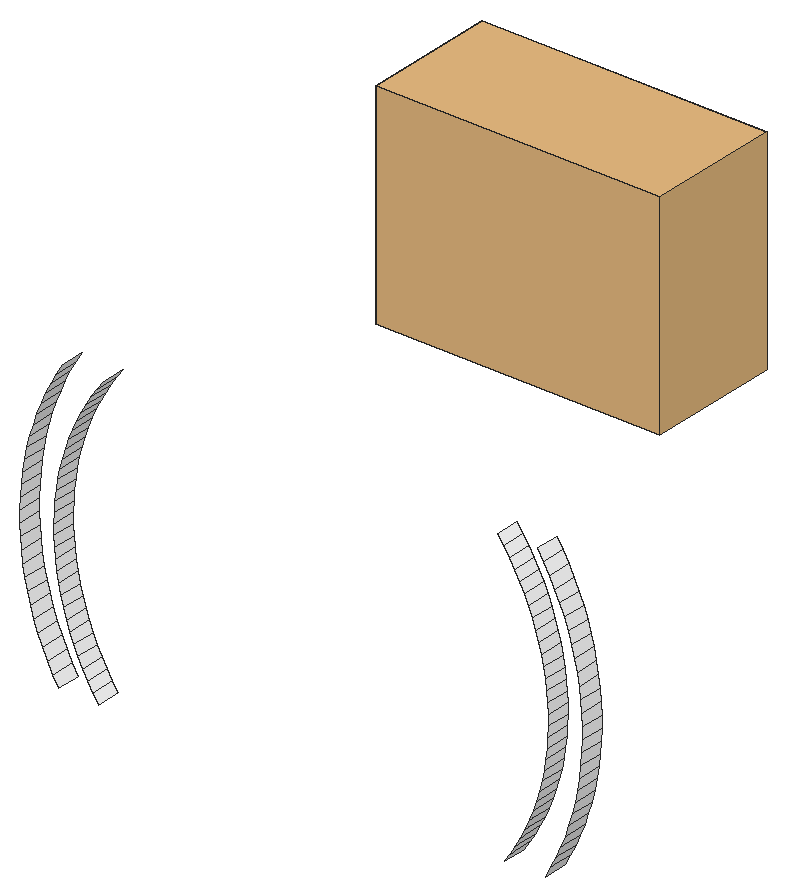
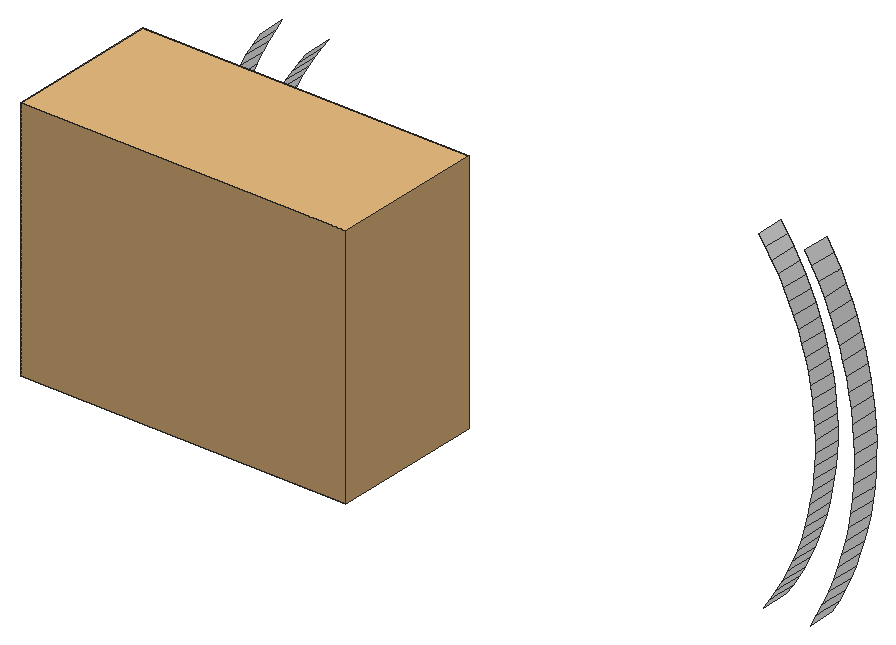
# SketchUp Ruby script. Lengths in inches.
U = 1.inch
M = Sketchup.active_model
def pt(a) = Geom::Point3d.new(a.map { |v| v * U })
def face(e, loops, mat)
  f = e.add_face(loops[0].map { |a| pt(a) })
  loops[1..].each { |l| e.add_face(l.map { |a| pt(a) }).erase! }
  f.material = f.back_material = mat if mat
  f
end
# faces: each face lists its corners as indices into pts; further lists are holes
def faces(e, pts, list, mat = nil) = list.each { |f| face(e, (f[0].is_a?(Array) ? f : [f]).map { |l| l.map { |i| pts[i] } }, mat) }
# xy, xz, yz: faces in a plane at the given z, y or x. An outline is a flat list of corners, or four numbers for a rectangle; further outlines are holes
def ring(l) = l.size == 4 ? [[l[0], l[1]], [l[2], l[1]], [l[2], l[3]], [l[0], l[3]]] : l.each_slice(2).to_a
def flat(e, list, mat, &to3) = list.each { |f| face(e, (f[0].is_a?(Array) ? f : [f]).map { |l| ring(l).map { |u, v| to3.(u, v) } }, mat) }
def xy(e, z, list, mat = nil) = flat(e, list, mat) { |x, y| [x, y, z] }
def xz(e, y, list, mat = nil) = flat(e, list, mat) { |x, z| [x, y, z] }
def yz(e, x, list, mat = nil) = flat(e, list, mat) { |y, z| [x, y, z] }
def lines(e, pts, list) = list.each { |a, b| e.add_line(pt(pts[a]), pt(pts[b])) }
# prism: a flat outline (further loops are holes) pulled along v
def prism(e, loops, v, mat = nil)
  f = face(e, loops, mat); d = Geom::Vector3d.new(v.map { |x| x * U })
  f.pushpull(f.normal.samedirection?(d) ? d.length : -d.length)
end
def box(e, o, s, mat = nil) = prism(e, [[o, [o[0] + s[0], o[1], o[2]], [o[0] + s[0], o[1] + s[1], o[2]], [o[0], o[1] + s[1], o[2]]]], [0, 0, s[2]], mat)
def at(x, y, z, deg = 0) = Geom::Transformation.translation(pt([x, y, z])) * Geom::Transformation.rotation(ORIGIN, Z_AXIS, deg.degrees)
def axes(o, x, y, z) = Geom::Transformation.new([*x, 0, *y, 0, *z, 0, *pt(o).to_a, 1])
def part(name) = M.definitions.add(name)
# library, detail: a bought-in or finely detailed component or shape, given as its bounding box
def library(name, o, s) = part(name).tap { |d| box(d.entities, o, s) }
def detail(e, o, s) = box(e.add_group.entities, o, s)
def put(e, d, t, mat = nil) = e.add_instance(d, t).tap { |i| i.material = mat if mat }
def group(e, t, mat = nil) = e.add_group.tap { |g| g.transformation = t; g.material = mat if mat }.entities
root = M.entities
M.materials.add("Leather White 002 15.0cm").color = [255, 255, 255]
c1 = library("Window Crafter Awning",[0,-9.5,0],[24,11.27,18])
yz(root,12.9,[[48.93,201.61,50.93,202.49]],"Leather White 002 15.0cm")
yz(root,57.52,[[48.93,201.78,50.93,202.77]],"Leather White 002 15.0cm")
p = [[12.79,50.93,191.04],[13.27,50.93,190.17],[13.27,48.93,190.17],[12.79,48.93,191.04],[16.69,50.93,190.15],[16.21,50.93,190.875],
  [16.21,48.93,190.875],[16.69,48.93,190.15],[51.47,50.93,191.06],[50.99,50.93,190.33],[50.99,48.93,190.33],[51.47,48.93,191.06],
  [54.41,50.93,190.39],[54.88,50.93,191.26],[54.88,48.93,191.26],[54.41,48.93,190.39],[15.75,50.93,191.62],[15.75,48.93,191.62],
  [12.34,50.93,191.93],[12.34,48.93,191.93],[51.91,50.93,191.81],[51.91,48.93,191.81],[55.32,50.93,192.15],[55.32,48.93,192.15],
  [15.32,50.93,192.39],[15.32,48.93,192.39],[52.33,50.93,192.58],[52.33,48.93,192.58],[11.93,50.93,192.84],[11.93,48.93,192.84],
  [55.72,50.93,193.0625],[55.72,48.93,193.0625],[14.93,50.93,193.17],[14.93,48.93,193.17],[52.72,50.93,193.36],[52.72,48.93,193.36],
  [11.56,50.93,193.76],[11.56,48.93,193.76],[56.08,50.93,193.99],[56.08,48.93,193.99],[14.57,50.93,193.96],[14.57,48.93,193.96],
  [53.07,50.93,194.16],[53.07,48.93,194.16],[11.23,50.93,194.7],[11.23,48.93,194.7],[14.24,50.93,194.78],[14.24,48.93,194.78],
  [56.4,50.93,194.93],[56.4,48.93,194.93],[53.39,50.93,194.98],[53.39,48.93,194.98],[10.9375,50.93,195.65],[10.9375,48.93,195.65],
  [13.95,50.93,195.6],[13.95,48.93,195.6],[56.69,50.93,195.89],[56.69,48.93,195.89],[53.67,50.93,195.8],[53.67,48.93,195.8],
  [13.7,50.93,196.4375],[13.7,48.93,196.4375],[10.68,50.93,196.61],[10.68,48.93,196.61],[53.92,50.93,196.64],[53.92,48.93,196.64],
  [56.93,50.93,196.85],[56.93,48.93,196.85],[13.47,50.93,197.28],[13.47,48.93,197.28],[10.47,50.93,197.59],[10.47,48.93,197.59],
  [54.13,50.93,197.49],[54.13,48.93,197.49],[57.13,50.93,197.82],[57.13,48.93,197.82],[13.29,50.93,198.14],[13.29,48.93,198.14],
  [54.31,50.93,198.35],[54.31,48.93,198.35],[10.3,50.93,198.57],[10.3,48.93,198.57],[57.29,50.93,198.81],[57.29,48.93,198.81],
  [13.14,50.93,199],[13.14,48.93,199],[54.45,50.93,199.21],[54.45,48.93,199.21],[10.17,50.93,199.55],[10.17,48.93,199.55],
  [57.41,50.93,199.79],[57.41,48.93,199.79],[13.02,50.93,199.87],[13.02,48.93,199.87],[54.56,50.93,200.08],[54.56,48.93,200.08],
  [10.08,50.93,200.54],[10.08,48.93,200.54],[57.49,50.93,200.79],[57.49,48.93,200.79],[12.95,50.93,200.74],[12.95,48.93,200.74],
  [54.625,50.93,200.95],[54.625,48.93,200.95],[10.04,50.93,201.54],[10.04,48.93,201.54],[12.9,50.93,201.61],[12.9,48.93,201.61],
  [57.52,50.93,201.78],[57.52,48.93,201.78],[54.66,50.93,201.83],[54.66,48.93,201.83],[10.03,50.93,202.53],[10.03,48.93,202.53],
  [54.65,50.93,202.7],[54.65,48.93,202.7],[10.07,50.93,203.52],[10.07,48.93,203.52],[12.9,50.93,202.49],[12.93,50.93,203.36],
  [12.93,48.93,203.36],[12.9,48.93,202.49],[54.61,50.93,203.57],[54.61,48.93,203.57],[57.52,50.93,202.77],[57.47,50.93,203.77],
  [57.47,48.93,203.77],[57.52,48.93,202.77],[13,50.93,204.23],[13,48.93,204.23],[10.15,50.93,204.52],[10.15,48.93,204.52],
  [54.53,50.93,204.44],[54.53,48.93,204.44],[57.38,50.93,204.76],[57.38,48.93,204.76],[13.11,50.93,205.1],[13.11,48.93,205.1],
  [54.42,50.93,205.3125],[54.42,48.93,205.3125],[10.27,50.93,205.5],[10.27,48.93,205.5],[57.25,50.93,205.75],[57.25,48.93,205.75],
  [13.25,50.93,205.96],[13.25,48.93,205.96],[54.27,50.93,206.17],[54.27,48.93,206.17],[10.43,50.93,206.49],[10.43,48.93,206.49],
  [57.08,50.93,206.73],[57.08,48.93,206.73],[13.42,50.93,206.82],[13.42,48.93,206.82],[54.08,50.93,207.03],[54.08,48.93,207.03],
  [10.63,50.93,207.46],[10.63,48.93,207.46],[56.87,50.93,207.7],[56.87,48.93,207.7],[13.64,50.93,207.67],[13.64,48.93,207.67],
  [53.86,50.93,207.875],[53.86,48.93,207.875],[10.87,50.93,208.42],[10.87,48.93,208.42],[13.89,50.93,208.51],[13.89,48.93,208.51],
  [56.62,50.93,208.66],[56.62,48.93,208.66],[53.6,50.93,208.71],[53.6,48.93,208.71],[11.15,50.93,209.38],[11.15,48.93,209.38],
  [14.17,50.93,209.33],[14.17,48.93,209.33],[53.3125,50.93,209.53],[53.3125,48.93,209.53],[56.33,50.93,209.61],[56.33,48.93,209.61],
  [14.49,50.93,210.15],[14.49,48.93,210.15],[11.48,50.93,210.32],[11.48,48.93,210.32],[52.99,50.93,210.35],[52.99,48.93,210.35],
  [56,50.93,210.55],[56,48.93,210.55],[14.84,50.93,210.95],[14.84,48.93,210.95],[11.84,50.93,211.25],[11.84,48.93,211.25],
  [52.625,50.93,211.14],[52.625,48.93,211.14],[55.625,50.93,211.47],[55.625,48.93,211.47],[15.22,50.93,211.73],[15.22,48.93,211.73],
  [52.23,50.93,211.92],[52.23,48.93,211.92],[12.24,50.93,212.16],[12.24,48.93,212.16],[55.22,50.93,212.38],[55.22,48.93,212.38],
  [15.64,50.93,212.5],[15.64,48.93,212.5],[51.81,50.93,212.6875],[51.81,48.93,212.6875],[12.67,50.93,213.05],[12.67,48.93,213.05],
  [54.77,50.93,213.27],[54.77,48.93,213.27],[16.09,50.93,213.25],[16.09,48.93,213.25],[51.35,50.93,213.43],[51.35,48.93,213.43],
  [13.15,50.93,213.92],[13.15,48.93,213.92],[16.57,50.93,213.98],[16.57,48.93,213.98],[54.28,50.93,214.14],[54.28,48.93,214.14],
  [50.86,50.93,214.16],[50.86,48.93,214.16],[13.66,50.93,214.78],[13.66,48.93,214.78],[17.08,50.93,214.69],[17.08,48.93,214.69],
  [53.77,50.93,214.98],[53.77,48.93,214.98],[50.35,50.93,214.87],[50.35,48.93,214.87]]
faces(root,p,[[0,1,2,3],[4,5,6,7],[8,9,10,11],[12,13,14,15],[5,16,17,6],[18,0,3,19],[20,8,11,21],[13,22,23,14],
  [16,24,25,17],[26,20,21,27],[28,18,19,29],[22,30,31,23],[24,32,33,25],[34,26,27,35],[36,28,29,37],[30,38,39,31],
  [32,40,41,33],[42,34,35,43],[44,36,37,45],[40,46,47,41],[38,48,49,39],[50,42,43,51],[52,44,45,53],[46,54,55,47],
  [48,56,57,49],[58,50,51,59],[54,60,61,55],[62,52,53,63],[64,58,59,65],[56,66,67,57],[60,68,69,61],[70,62,63,71],
  [72,64,65,73],[66,74,75,67],[68,76,77,69],[78,72,73,79],[80,70,71,81],[74,82,83,75],[76,84,85,77],[86,78,79,87],
  [88,80,81,89],[82,90,91,83],[84,92,93,85],[94,86,87,95],[96,88,89,97],[90,98,99,91],[92,100,101,93],[102,94,95,103],
  [104,96,97,105],[100,106,107,101],[98,108,109,99],[110,102,103,111],[112,104,105,113],[114,110,111,115],[116,112,113,117],[118,119,120,121],
  [122,114,115,123],[124,125,126,127],[119,128,129,120],[130,116,117,131],[132,122,123,133],[125,134,135,126],[128,136,137,129],[138,132,133,139],
  [140,130,131,141],[134,142,143,135],[136,144,145,137],[146,138,139,147],[148,140,141,149],[142,150,151,143],[144,152,153,145],[154,146,147,155],
  [156,148,149,157],[150,158,159,151],[152,160,161,153],[162,154,155,163],[164,156,157,165],[160,166,167,161],[158,168,169,159],[170,162,163,171],
  [172,164,165,173],[166,174,175,167],[176,170,171,177],[168,178,179,169],[174,180,181,175],[182,172,173,183],[184,176,177,185],[178,186,187,179],
  [180,188,189,181],[190,182,183,191],[192,184,185,193],[186,194,195,187],[188,196,197,189],[198,192,193,199],[200,190,191,201],[194,202,203,195],
  [196,204,205,197],[206,198,199,207],[208,200,201,209],[202,210,211,203],[204,212,213,205],[214,206,207,215],[216,208,209,217],[212,218,219,213],
  [210,220,221,211],[222,214,215,223],[224,216,217,225],[218,226,227,219],[220,228,229,221],[230,222,223,231]],"Leather White 002 15.0cm")
put(root,c1,at(21,82.23,210))
